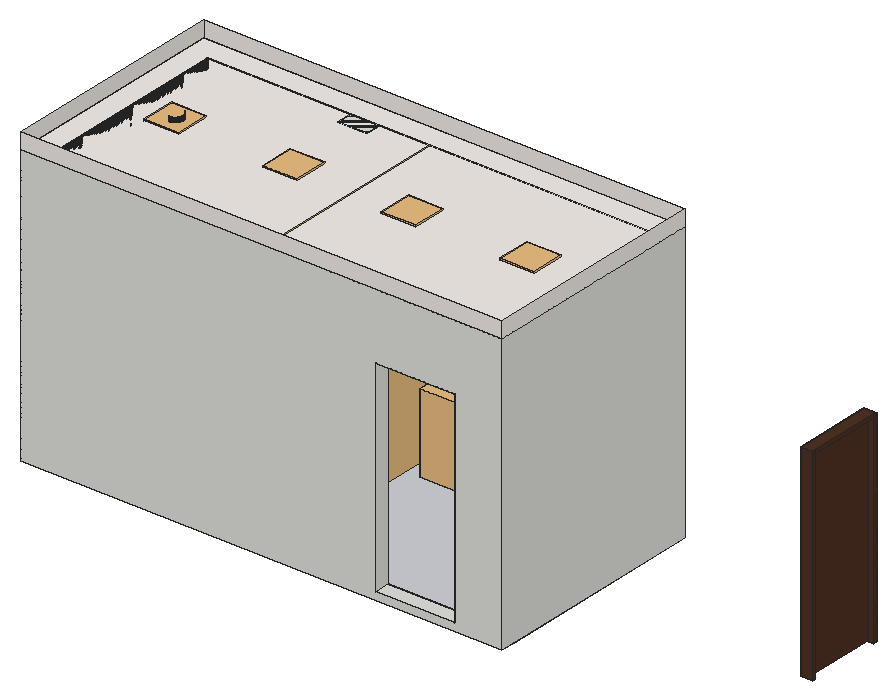
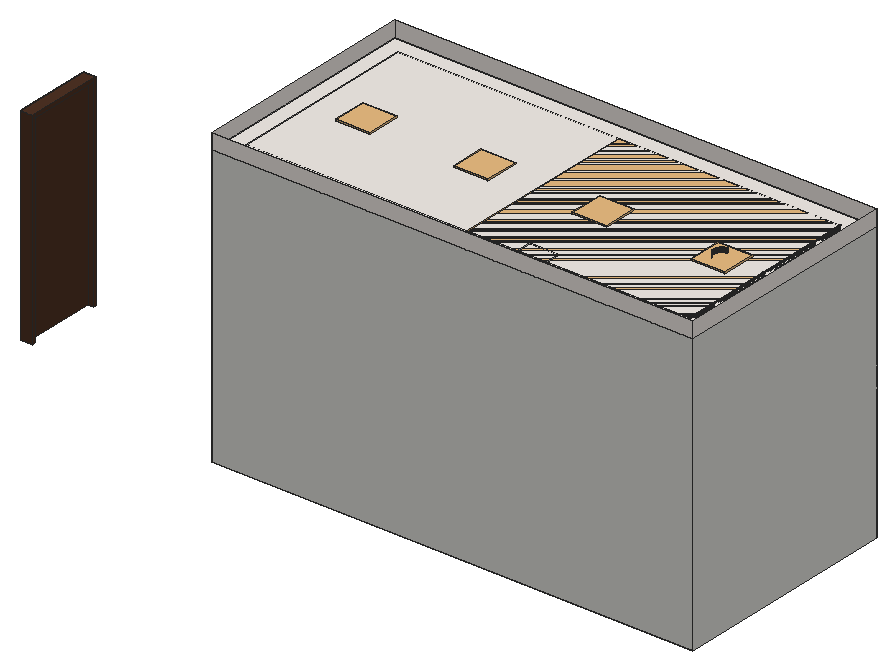
# SketchUp Ruby script. Lengths in inches.
U = 1.inch
M = Sketchup.active_model
def pt(a) = Geom::Point3d.new(a.map { |v| v * U })
def face(e, loops, mat)
  f = e.add_face(loops[0].map { |a| pt(a) })
  loops[1..].each { |l| e.add_face(l.map { |a| pt(a) }).erase! }
  f.material = f.back_material = mat if mat
  f
end
# faces: each face lists its corners as indices into pts; further lists are holes
def faces(e, pts, list, mat = nil) = list.each { |f| face(e, (f[0].is_a?(Array) ? f : [f]).map { |l| l.map { |i| pts[i] } }, mat) }
# xy, xz, yz: faces in a plane at the given z, y or x. An outline is a flat list of corners, or four numbers for a rectangle; further outlines are holes
def ring(l) = l.size == 4 ? [[l[0], l[1]], [l[2], l[1]], [l[2], l[3]], [l[0], l[3]]] : l.each_slice(2).to_a
def flat(e, list, mat, &to3) = list.each { |f| face(e, (f[0].is_a?(Array) ? f : [f]).map { |l| ring(l).map { |u, v| to3.(u, v) } }, mat) }
def xy(e, z, list, mat = nil) = flat(e, list, mat) { |x, y| [x, y, z] }
def xz(e, y, list, mat = nil) = flat(e, list, mat) { |x, z| [x, y, z] }
def yz(e, x, list, mat = nil) = flat(e, list, mat) { |y, z| [x, y, z] }
def lines(e, pts, list) = list.each { |a, b| e.add_line(pt(pts[a]), pt(pts[b])) }
# prism: a flat outline (further loops are holes) pulled along v
def prism(e, loops, v, mat = nil)
  f = face(e, loops, mat); d = Geom::Vector3d.new(v.map { |x| x * U })
  f.pushpull(f.normal.samedirection?(d) ? d.length : -d.length)
end
def box(e, o, s, mat = nil) = prism(e, [[o, [o[0] + s[0], o[1], o[2]], [o[0] + s[0], o[1] + s[1], o[2]], [o[0], o[1] + s[1], o[2]]]], [0, 0, s[2]], mat)
def at(x, y, z, deg = 0) = Geom::Transformation.translation(pt([x, y, z])) * Geom::Transformation.rotation(ORIGIN, Z_AXIS, deg.degrees)
def axes(o, x, y, z) = Geom::Transformation.new([*x, 0, *y, 0, *z, 0, *pt(o).to_a, 1])
def part(name) = M.definitions.add(name)
# library, detail: a bought-in or finely detailed component or shape, given as its bounding box
def library(name, o, s) = part(name).tap { |d| box(d.entities, o, s) }
def detail(e, o, s) = box(e.add_group.entities, o, s)
def put(e, d, t, mat = nil) = e.add_instance(d, t).tap { |i| i.material = mat if mat }
def group(e, t, mat = nil) = e.add_group.tap { |g| g.transformation = t; g.material = mat if mat }.entities
root = M.entities
M.materials.add("0001 AP 9436 AIR BREEZE").color = [243, 237, 232]
M.materials.add("Polis06_194").color = [79, 50, 36]
M.materials.add("Shelves Light").color = [253, 215, 186]
M.materials.add("[Color M00]").color = [255, 255, 255]
M.materials.add("[Marble Carrara Floor Tile]").color = [207, 209, 215]
M.materials.add("[Stone Vein Gray]").color = [234, 229, 229]
M.materials.add("[Terrazzo Tile Light]").color = [219, 217, 210]
c1 = library("Bathrobe with hooks",[0,0,-0.08],[18.125,10.02,52.34])
c2 = library("Bathroom toiletries",[0,-0.3,0],[24.27,4.3,11.74])
c3 = library("Basket & Towel",[-7.51,-8.15,0],[15.02,16.3,23.9375])
c4 = library("JEE-O slimline shower set bronze\#1",[0.04,-0.03,-18.98],[11.61,24.11,65.69])
c5 = library("Group\#4",[-0.25,-72,0],[84.37,72,106])
c6 = part("Difference1")
box(c6.entities,[0,-6,0],[11,6,100])
c7 = part("2")
prism(c7.entities,[[[0.125,0,0],[0.25,0,0],[0.25,0,0.02],[0.25,0,0.03],[0.24,0,0.05],[0.23,0,0.0625],[0.22,0,0.08],[0.21,0,0.09],[0.2,0,0.1],[0.1875,0,0.11],[0.17,0,0.12],[0.16,0,0.12],[0.14,0,0.125],[0.125,0,0.125],[0.11,0,0.125],[0.09,0,0.12],[0.08,0,0.12],[0.0625,0,0.11],[0.05,0,0.1],[0.04,0,0.09],[0.03,0,0.08],[0.02,0,0.0625],[0.01,0,0.05],[0,0,0.03],[0,0,0.02],[0,0,0]]],[0,18,0])
c8 = part("Group\#11")
box(c8.entities,[0,0,0],[17,18,0.125])
g1 = group(c8.entities,at(0,0,0.125))
put(g1,c7,at(2.0625,0,0))
put(g1,c7,at(9.53,0,0))
put(g1,c7,at(10.05,0,0))
put(g1,c7,at(10.57,0,0))
put(g1,c7,at(10.82,0,0))
put(g1,c7,at(5.67,0,0))
put(g1,c7,at(2.32,0,0))
put(g1,c7,at(3.09,0,0))
put(g1,c7,at(1.03,0,0))
put(g1,c7,at(0.77,0,0))
put(g1,c7,at(3.35,0,0))
put(g1,c7,at(5.15,0,0))
put(g1,c7,at(4.38,0,0))
put(g1,c7,at(7.47,0,0))
put(g1,c7,at(8.5,0,0))
put(g1,c7,at(10.31,0,0))
put(g1,c7,at(11.08,0,0))
put(g1,c7,at(2.83,0,0))
put(g1,c7,at(0,0,0))
put(g1,c7,at(1.55,0,0))
put(g1,c7,at(4.125,0,0))
put(g1,c7,at(4.64,0,0))
put(g1,c7,at(4.9,0,0))
put(g1,c7,at(5.41,0,0))
put(g1,c7,at(8.76,0,0))
put(g1,c7,at(3.61,0,0))
put(g1,c7,at(0.52,0,0))
put(g1,c7,at(6.96,0,0))
put(g1,c7,at(7.22,0,0))
put(g1,c7,at(1.29,0,0))
put(g1,c7,at(6.44,0,0))
put(g1,c7,at(7.73,0,0))
put(g1,c7,at(2.58,0,0))
put(g1,c7,at(3.87,0,0))
put(g1,c7,at(6.18,0,0))
put(g1,c7,at(8.25,0,0))
put(g1,c7,at(6.7,0,0))
put(g1,c7,at(9.02,0,0))
put(g1,c7,at(9.79,0,0))
put(g1,c7,at(0.26,0,0))
put(g1,c7,at(1.8,0,0))
put(g1,c7,at(9.28,0,0))
put(g1,c7,at(5.93,0,0))
put(g1,c7,at(7.99,0,0))
put(g1,c7,at(13.92,0,0))
put(g1,c7,at(14.43,0,0))
put(g1,c7,at(14.6875,0,0))
put(g1,c7,at(13.4,0,0))
put(g1,c7,at(12.625,0,0))
put(g1,c7,at(15.98,0,0))
put(g1,c7,at(11.6,0,0))
put(g1,c7,at(11.34,0,0))
put(g1,c7,at(12.88,0,0))
put(g1,c7,at(11.85,0,0))
put(g1,c7,at(13.66,0,0))
put(g1,c7,at(15.2,0,0))
put(g1,c7,at(15.72,0,0))
put(g1,c7,at(14.17,0,0))
put(g1,c7,at(14.95,0,0))
put(g1,c7,at(12.11,0,0))
put(g1,c7,at(12.37,0,0))
put(g1,c7,at(16.23,0,0))
put(g1,c7,at(13.14,0,0))
put(g1,c7,at(16.75,0,0))
put(g1,c7,at(16.49,0,0))
put(g1,c7,at(15.46,0,0))
c9 = part("Group\#9")
put(c9.entities,c8,at(0,0,0.25))
c10 = part("Group\#5")
put(c10.entities,c8,at(0,0,0.25))
c11 = part("Group\#13")
put(c11.entities,c8,at(0,0,0.25))
c12 = library("Group\#22",[0,-21,-2],[57,21,30])
c13 = part("Group\#28")
box(c13.entities,[0,0,-0.5],[18,1,0.5])
c14 = library("Group\#25",[0,-0.44,0],[39,1.19,41])
c15 = part("Bathroom door")
xy(c15.entities,0,[[0,0,4.72,1.18],[0,34.25,4.72,35.43]],"Polis06_194")
xy(c15.entities,85.26,[[0,1.18,4.72,34.25]],"Polis06_194")
xy(c15.entities,86.61,[[0,0,4.72,35.43]],"Polis06_194")
xz(c15.entities,0,[[0,0,4.72,86.61]],"Polis06_194")
xz(c15.entities,1.18,[[0,0,2.36,85.26],[2.36,0,4.72,85.26]],"Polis06_194")
xz(c15.entities,34.25,[[0,0,4.72,85.26]],"Polis06_194")
xz(c15.entities,35.43,[[0,0,4.72,86.61]],"Polis06_194")
yz(c15.entities,0,[[0,0,1.18,86.61],[34.25,0,35.43,86.61],[1.18,85.26,34.25,86.61]],"Polis06_194")
yz(c15.entities,2.36,[[1.18,0,34.25,0,34.25,85.21,1.18,85.26]],"Polis06_194")
yz(c15.entities,4.72,[[0,0,1.18,86.61],[34.25,0,35.43,86.61],[1.18,85.26,34.25,86.61]],"Polis06_194")
c16 = library("Health Faucet",[-0.24,3.23,-9.93],[3.46,9,32.04])
c17 = library("Cesto com toalhas",[0,-0.02,0],[20.47,20.49,27.38])
c18 = library("towels 1",[11.44,13.74,0],[9.37,7.5,4.04])
c19 = library("N_Bathroom Accessory 1",[-8.74,-6.98,-0.07],[10.13,6.73,7.64])
c20 = library("model 1",[0,0,0],[7.72,6.97,5.65])
c21 = library("Plant pots 03",[-13.35,-27.09,0],[26.22,40.73,41.57])
c22 = library("TowelAndHanger",[-0.24,-1.14,-0.4],[8.64,6.67,18.87])
c23 = library("Group\#46",[-1.6,-2.17,0],[14.44,14.68,15.07])
c24 = library("skp31A6",[-6.04,-1.48,32.125],[7.16,7.43,5.2])
c25 = library("Group\#73",[0,0,0],[5.51,2.625,8.11])
c26 = library("_CAPIM_DOS_PAMPAS_JULIAAIRES.3D",[-3.51,-2.78,-196.14],[35.86,35.18,43.25])
c27 = library("Group3\#1",[-226.43,63.68,0],[21.09,21.08,29.58])
c28 = library("15",[-4.61,-4.61,-12.23],[13.01,13.01,12.23])
xy(root,106,[[[0,0,183,87],[68.91,40.5,69.14,40.5,69.22,40.51,69.3,40.51,69.45,40.53,69.53,40.55,69.61,40.5625,69.84,40.62,69.91,40.64,69.99,40.67,70.06,40.69,70.13,40.72,70.21,40.75,70.28,40.79,70.35,40.82,70.42,40.86,70.49,40.89,70.55,40.93,70.62,40.98,70.6875,41.02,70.75,41.0625,70.8125,41.11,71,41.26,71.05,41.3125,71.11,41.37,71.22,41.48,71.42,41.72,71.46,41.79,71.51,41.85,71.59,41.99,71.63,42.05,71.67,42.125,71.7,42.19,71.73,42.26,71.77,42.34,71.79,42.41,71.82,42.48,71.85,42.56,71.87,42.63,71.89,42.71,71.91,42.78,71.93,42.86,71.95,42.9375,71.96,43.01,71.99,43.25,71.99,43.33,72,43.41,72,43.64,71.99,43.72,71.99,43.8,71.97,43.95,71.95,44.03,71.9375,44.11,71.88,44.34,71.86,44.41,71.83,44.49,71.81,44.56,71.78,44.63,71.75,44.71,71.71,44.78,71.68,44.85,71.64,44.92,71.61,44.99,71.57,45.05,71.52,45.12,71.48,45.1875,71.4375,45.25,71.39,45.3125,71.24,45.5,71.1875,45.55,71.13,45.61,71.02,45.72,70.78,45.92,70.71,45.96,70.65,46.01,70.51,46.09,70.45,46.13,70.375,46.17,70.31,46.2,70.24,46.23,70.16,46.27,70.09,46.29,70.02,46.32,69.94,46.35,69.87,46.37,69.79,46.39,69.72,46.41,69.64,46.43,69.5625,46.45,69.49,46.46,69.25,46.49,69.17,46.49,69.09,46.5,68.86,46.5,68.78,46.49,68.7,46.49,68.55,46.47,68.47,46.45,68.39,46.4375,68.16,46.38,68.09,46.36,68.01,46.33,67.94,46.31,67.87,46.28,67.79,46.25,67.72,46.21,67.65,46.18,67.58,46.14,67.51,46.11,67.45,46.07,67.38,46.02,67.3125,45.98,67.25,45.9375,67.1875,45.89,67,45.74,66.95,45.6875,66.89,45.63,66.78,45.52,66.58,45.28,66.54,45.21,66.49,45.15,66.41,45.01,66.37,44.95,66.33,44.875,66.3,44.81,66.27,44.74,66.23,44.66,66.21,44.59,66.18,44.52,66.15,44.44,66.13,44.37,66.11,44.29,66.09,44.22,66.07,44.14,66.05,44.0625,66.04,43.99,66.01,43.75,66.01,43.67,66,43.59,66,43.36,66.01,43.28,66.01,43.2,66.03,43.05,66.05,42.97,66.0625,42.89,66.12,42.66,66.14,42.59,66.17,42.51,66.19,42.44,66.22,42.37,66.25,42.29,66.29,42.22,66.32,42.15,66.36,42.08,66.39,42.01,66.43,41.95,66.48,41.88,66.52,41.8125,66.5625,41.75,66.61,41.6875,66.76,41.5,66.8125,41.45,66.87,41.39,66.98,41.28,67.22,41.08,67.29,41.04,67.35,40.99,67.49,40.91,67.55,40.87,67.625,40.83,67.69,40.8,67.76,40.77,67.84,40.73,67.91,40.71,67.98,40.68,68.06,40.65,68.13,40.63,68.21,40.61,68.28,40.59,68.36,40.57,68.4375,40.55,68.51,40.54,68.75,40.51,68.83,40.51],[23.91,40.5,24.14,40.5,24.22,40.51,24.3,40.51,24.45,40.53,24.53,40.55,24.61,40.5625,24.84,40.62,24.91,40.64,24.99,40.67,25.06,40.69,25.13,40.72,25.21,40.75,25.28,40.79,25.35,40.82,25.42,40.86,25.49,40.89,25.55,40.93,25.62,40.98,25.6875,41.02,25.75,41.0625,25.8125,41.11,26,41.26,26.05,41.3125,26.11,41.37,26.22,41.48,26.42,41.72,26.46,41.79,26.51,41.85,26.59,41.99,26.63,42.05,26.67,42.125,26.7,42.19,26.73,42.26,26.77,42.34,26.79,42.41,26.82,42.48,26.85,42.56,26.87,42.63,26.89,42.71,26.91,42.78,26.93,42.86,26.95,42.9375,26.96,43.01,26.99,43.25,26.99,43.33,27,43.41,27,43.64,26.99,43.72,26.99,43.8,26.97,43.95,26.95,44.03,26.9375,44.11,26.88,44.34,26.86,44.41,26.83,44.49,26.81,44.56,26.78,44.63,26.75,44.71,26.71,44.78,26.68,44.85,26.64,44.92,26.61,44.99,26.57,45.05,26.52,45.12,26.48,45.1875,26.4375,45.25,26.39,45.3125,26.24,45.5,26.1875,45.55,26.13,45.61,26.02,45.72,25.78,45.92,25.71,45.96,25.65,46.01,25.51,46.09,25.45,46.13,25.375,46.17,25.31,46.2,25.24,46.23,25.16,46.27,25.09,46.29,25.02,46.32,24.94,46.35,24.87,46.37,24.79,46.39,24.72,46.41,24.64,46.43,24.5625,46.45,24.49,46.46,24.25,46.49,24.17,46.49,24.09,46.5,23.86,46.5,23.78,46.49,23.7,46.49,23.55,46.47,23.47,46.45,23.39,46.4375,23.16,46.38,23.09,46.36,23.01,46.33,22.94,46.31,22.87,46.28,22.79,46.25,22.72,46.21,22.65,46.18,22.58,46.14,22.51,46.11,22.45,46.07,22.38,46.02,22.3125,45.98,22.25,45.9375,22.1875,45.89,22,45.74,21.95,45.6875,21.89,45.63,21.78,45.52,21.58,45.28,21.54,45.21,21.49,45.15,21.41,45.01,21.37,44.95,21.33,44.875,21.3,44.81,21.27,44.74,21.23,44.66,21.21,44.59,21.18,44.52,21.15,44.44,21.13,44.37,21.11,44.29,21.09,44.22,21.07,44.14,21.05,44.0625,21.04,43.99,21.01,43.75,21.01,43.67,21,43.59,21,43.36,21.01,43.28,21.01,43.2,21.03,43.05,21.05,42.97,21.0625,42.89,21.12,42.66,21.14,42.59,21.17,42.51,21.19,42.44,21.22,42.37,21.25,42.29,21.29,42.22,21.32,42.15,21.36,42.08,21.39,42.01,21.43,41.95,21.48,41.88,21.52,41.8125,21.5625,41.75,21.61,41.6875,21.76,41.5,21.8125,41.45,21.87,41.39,21.98,41.28,22.22,41.08,22.29,41.04,22.35,40.99,22.49,40.91,22.55,40.87,22.625,40.83,22.69,40.8,22.76,40.77,22.84,40.73,22.91,40.71,22.98,40.68,23.06,40.65,23.13,40.63,23.21,40.61,23.28,40.59,23.36,40.57,23.4375,40.55,23.51,40.54,23.75,40.51,23.83,40.51],[158.91,40.5,159.14,40.5,159.22,40.51,159.3,40.51,159.45,40.53,159.53,40.55,159.61,40.5625,159.84,40.62,159.91,40.64,159.99,40.67,160.06,40.69,160.13,40.72,160.21,40.75,160.28,40.79,160.35,40.82,160.42,40.86,160.49,40.89,160.55,40.93,160.62,40.98,160.6875,41.02,160.75,41.0625,160.8125,41.11,161,41.26,161.05,41.3125,161.11,41.37,161.22,41.48,161.42,41.72,161.46,41.79,161.51,41.85,161.59,41.99,161.63,42.05,161.67,42.125,161.7,42.19,161.73,42.26,161.77,42.34,161.79,42.41,161.82,42.48,161.85,42.56,161.87,42.63,161.89,42.71,161.91,42.78,161.93,42.86,161.95,42.9375,161.96,43.01,161.99,43.25,161.99,43.33,162,43.41,162,43.64,161.99,43.72,161.99,43.8,161.97,43.95,161.95,44.03,161.9375,44.11,161.88,44.34,161.86,44.41,161.83,44.49,161.81,44.56,161.78,44.63,161.75,44.71,161.71,44.78,161.68,44.85,161.64,44.92,161.61,44.99,161.57,45.05,161.52,45.12,161.48,45.1875,161.4375,45.25,161.39,45.3125,161.24,45.5,161.1875,45.55,161.13,45.61,161.02,45.72,160.78,45.92,160.71,45.96,160.65,46.01,160.51,46.09,160.45,46.13,160.375,46.17,160.31,46.2,160.24,46.23,160.16,46.27,160.09,46.29,160.02,46.32,159.94,46.35,159.87,46.37,159.79,46.39,159.72,46.41,159.64,46.43,159.5625,46.45,159.49,46.46,159.25,46.49,159.17,46.49,159.09,46.5,158.86,46.5,158.78,46.49,158.7,46.49,158.55,46.47,158.47,46.45,158.39,46.4375,158.16,46.38,158.09,46.36,158.01,46.33,157.94,46.31,157.87,46.28,157.79,46.25,157.72,46.21,157.65,46.18,157.58,46.14,157.51,46.11,157.45,46.07,157.38,46.02,157.3125,45.98,157.25,45.9375,157.1875,45.89,157,45.74,156.95,45.6875,156.89,45.63,156.78,45.52,156.58,45.28,156.54,45.21,156.49,45.15,156.41,45.01,156.37,44.95,156.33,44.875,156.3,44.81,156.27,44.74,156.23,44.66,156.21,44.59,156.18,44.52,156.15,44.44,156.13,44.37,156.11,44.29,156.09,44.22,156.07,44.14,156.05,44.0625,156.04,43.99,156.01,43.75,156.01,43.67,156,43.59,156,43.36,156.01,43.28,156.01,43.2,156.03,43.05,156.05,42.97,156.0625,42.89,156.12,42.66,156.14,42.59,156.17,42.51,156.19,42.44,156.22,42.37,156.25,42.29,156.29,42.22,156.32,42.15,156.36,42.08,156.39,42.01,156.43,41.95,156.48,41.88,156.52,41.8125,156.5625,41.75,156.61,41.6875,156.76,41.5,156.8125,41.45,156.87,41.39,156.98,41.28,157.22,41.08,157.29,41.04,157.35,40.99,157.49,40.91,157.55,40.87,157.625,40.83,157.69,40.8,157.76,40.77,157.84,40.73,157.91,40.71,157.98,40.68,158.06,40.65,158.13,40.63,158.21,40.61,158.28,40.59,158.36,40.57,158.4375,40.55,158.51,40.54,158.75,40.51,158.83,40.51],[113.91,40.5,114.14,40.5,114.22,40.51,114.3,40.51,114.45,40.53,114.53,40.55,114.61,40.5625,114.84,40.62,114.91,40.64,114.99,40.67,115.06,40.69,115.13,40.72,115.21,40.75,115.28,40.79,115.35,40.82,115.42,40.86,115.49,40.89,115.55,40.93,115.62,40.98,115.6875,41.02,115.75,41.0625,115.8125,41.11,116,41.26,116.05,41.3125,116.11,41.37,116.22,41.48,116.42,41.72,116.46,41.79,116.51,41.85,116.59,41.99,116.63,42.05,116.67,42.125,116.7,42.19,116.73,42.26,116.77,42.34,116.79,42.41,116.82,42.48,116.85,42.56,116.87,42.63,116.89,42.71,116.91,42.78,116.93,42.86,116.95,42.9375,116.96,43.01,116.99,43.25,116.99,43.33,117,43.41,117,43.64,116.99,43.72,116.99,43.8,116.97,43.95,116.95,44.03,116.9375,44.11,116.88,44.34,116.86,44.41,116.83,44.49,116.81,44.56,116.78,44.63,116.75,44.71,116.71,44.78,116.68,44.85,116.64,44.92,116.61,44.99,116.57,45.05,116.52,45.12,116.48,45.1875,116.4375,45.25,116.39,45.3125,116.24,45.5,116.1875,45.55,116.13,45.61,116.02,45.72,115.78,45.92,115.71,45.96,115.65,46.01,115.51,46.09,115.45,46.13,115.375,46.17,115.31,46.2,115.24,46.23,115.16,46.27,115.09,46.29,115.02,46.32,114.94,46.35,114.87,46.37,114.79,46.39,114.72,46.41,114.64,46.43,114.5625,46.45,114.49,46.46,114.25,46.49,114.17,46.49,114.09,46.5,113.86,46.5,113.78,46.49,113.7,46.49,113.55,46.47,113.47,46.45,113.39,46.4375,113.16,46.38,113.09,46.36,113.01,46.33,112.94,46.31,112.87,46.28,112.79,46.25,112.72,46.21,112.65,46.18,112.58,46.14,112.51,46.11,112.45,46.07,112.38,46.02,112.3125,45.98,112.25,45.9375,112.1875,45.89,112,45.74,111.95,45.6875,111.89,45.63,111.78,45.52,111.58,45.28,111.54,45.21,111.49,45.15,111.41,45.01,111.37,44.95,111.33,44.875,111.3,44.81,111.27,44.74,111.23,44.66,111.21,44.59,111.18,44.52,111.15,44.44,111.13,44.37,111.11,44.29,111.09,44.22,111.07,44.14,111.05,44.0625,111.04,43.99,111.01,43.75,111.01,43.67,111,43.59,111,43.36,111.01,43.28,111.01,43.2,111.03,43.05,111.05,42.97,111.0625,42.89,111.12,42.66,111.14,42.59,111.17,42.51,111.19,42.44,111.22,42.37,111.25,42.29,111.29,42.22,111.32,42.15,111.36,42.08,111.39,42.01,111.43,41.95,111.48,41.88,111.52,41.8125,111.5625,41.75,111.61,41.6875,111.76,41.5,111.8125,41.45,111.87,41.39,111.98,41.28,112.22,41.08,112.29,41.04,112.35,40.99,112.49,40.91,112.55,40.87,112.625,40.83,112.69,40.8,112.76,40.77,112.84,40.73,112.91,40.71,112.98,40.68,113.06,40.65,113.13,40.63,113.21,40.61,113.28,40.59,113.36,40.57,113.4375,40.55,113.51,40.54,113.75,40.51,113.83,40.51]]],"0001 AP 9436 AIR BREEZE")
xz(root,0,[[0,106,183,112]],"0001 AP 9436 AIR BREEZE")
xz(root,40.5,[[23.91,106,23.98,108],[23.98,106,24.0625,108],[24.0625,106,24.14,108]],"0001 AP 9436 AIR BREEZE")
xz(root,40.51,[[24.22,106,24.3,108]],"0001 AP 9436 AIR BREEZE")
xz(root,87,[[0,106,183,112]],"0001 AP 9436 AIR BREEZE")
yz(root,0,[[0,106,87,112]],"0001 AP 9436 AIR BREEZE")
yz(root,26.99,[[43.25,106,43.33,108],[43.72,106,43.8,108]],"0001 AP 9436 AIR BREEZE")
yz(root,27,[[43.41,106,43.48,108],[43.48,106,43.5625,108],[43.5625,106,43.64,108]],"0001 AP 9436 AIR BREEZE")
yz(root,183,[[0,106,87,112]],"0001 AP 9436 AIR BREEZE")
p = [[24.22,40.51,106],[24.14,40.5,106],[24.14,40.5,108],[24.22,40.51,108],[24.375,40.52,106],[24.3,40.51,106],
  [24.3,40.51,108],[24.375,40.52,108],[24.45,40.53,106],[24.45,40.53,108],[24.61,40.5625,106],[24.53,40.55,106],
  [24.53,40.55,108],[24.61,40.5625,108],[24.68,40.58,106],[24.68,40.58,108],[24.76,40.6,106],[24.76,40.6,108],
  [24.91,40.64,106],[24.84,40.62,106],[24.84,40.62,108],[24.91,40.64,108],[24.99,40.67,106],[24.99,40.67,108],
  [25.06,40.69,106],[25.06,40.69,108],[25.21,40.75,106],[25.13,40.72,106],[25.13,40.72,108],[25.21,40.75,108],
  [25.28,40.79,106],[25.28,40.79,108],[25.42,40.86,106],[25.35,40.82,106],[25.35,40.82,108],[25.42,40.86,108],
  [25.49,40.89,106],[25.49,40.89,108],[25.55,40.93,106],[25.55,40.93,108],[25.62,40.98,106],[25.62,40.98,108],
  [25.6875,41.02,106],[25.6875,41.02,108],[25.75,41.0625,106],[25.75,41.0625,108],[25.875,41.16,106],[25.8125,41.11,106],
  [25.8125,41.11,108],[25.875,41.16,108],[26,41.26,106],[25.9375,41.21,106],[25.9375,41.21,108],[26,41.26,108],
  [26.05,41.3125,106],[26.05,41.3125,108],[26.11,41.37,106],[26.11,41.37,108],[26.16,41.42,106],[26.16,41.42,108],
  [26.22,41.48,106],[26.22,41.48,108],[26.27,41.54,106],[26.27,41.54,108],[26.32,41.6,106],[26.32,41.6,108],
  [26.37,41.66,106],[26.37,41.66,108],[26.46,41.79,106],[26.42,41.72,106],[26.42,41.72,108],[26.46,41.79,108],
  [26.51,41.85,106],[26.51,41.85,108],[26.59,41.99,106],[26.55,41.92,106],[26.55,41.92,108],[26.59,41.99,108],
  [26.63,42.05,106],[26.63,42.05,108],[26.67,42.125,106],[26.67,42.125,108],[26.7,42.19,106],[26.7,42.19,108],
  [26.73,42.26,106],[26.73,42.26,108],[26.77,42.34,106],[26.77,42.34,108],[26.79,42.41,106],[26.79,42.41,108],
  [26.82,42.48,106],[26.82,42.48,108],[26.85,42.56,106],[26.85,42.56,108],[26.87,42.63,106],[26.87,42.63,108],
  [26.89,42.71,106],[26.89,42.71,108],[26.91,42.78,106],[26.91,42.78,108],[26.93,42.86,106],[26.93,42.86,108],
  [26.96,43.01,106],[26.95,42.9375,106],[26.95,42.9375,108],[26.96,43.01,108],[26.97,43.09,106],[26.97,43.09,108],
  [26.98,43.17,106],[26.98,43.17,108],[26.99,43.25,106],[26.99,43.25,108],[27,43.41,106],[26.99,43.33,106],
  [26.99,43.33,108],[27,43.41,108],[26.99,43.72,106],[27,43.64,106],[27,43.64,108],[26.99,43.72,108],
  [26.98,43.875,106],[26.99,43.8,106],[26.99,43.8,108],[26.98,43.875,108],[26.97,43.95,106],[26.97,43.95,108],
  [26.9375,44.11,106],[26.95,44.03,106],[26.95,44.03,108],[26.9375,44.11,108],[26.92,44.18,106],[26.92,44.18,108],
  [26.9,44.26,106],[26.9,44.26,108],[26.86,44.41,106],[26.88,44.34,106],[26.88,44.34,108],[26.86,44.41,108],
  [26.83,44.49,106],[26.83,44.49,108],[26.81,44.56,106],[26.81,44.56,108],[26.75,44.71,106],[26.78,44.63,106],
  [26.78,44.63,108],[26.75,44.71,108],[26.71,44.78,106],[26.71,44.78,108],[26.64,44.92,106],[26.68,44.85,106],
  [26.68,44.85,108],[26.64,44.92,108],[26.61,44.99,106],[26.61,44.99,108],[26.57,45.05,106],[26.57,45.05,108],
  [26.48,45.1875,106],[26.52,45.12,106],[26.52,45.12,108],[26.48,45.1875,108],[26.4375,45.25,106],[26.4375,45.25,108],
  [26.34,45.375,106],[26.39,45.3125,106],[26.39,45.3125,108],[26.34,45.375,108],[26.24,45.5,106],[26.29,45.4375,106],
  [26.29,45.4375,108],[26.24,45.5,108],[26.1875,45.55,106],[26.1875,45.55,108],[26.08,45.66,106],[26.13,45.61,106],
  [26.13,45.61,108],[26.08,45.66,108],[25.96,45.77,106],[26.02,45.72,106],[26.02,45.72,108],[25.96,45.77,108],
  [25.84,45.87,106],[25.9,45.82,106],[25.9,45.82,108],[25.84,45.87,108],[25.78,45.92,106],[25.78,45.92,108]]
faces(root,p,[[0,1,2,3],[4,5,6,7],[8,4,7,9],[10,11,12,13],[11,8,9,12],[14,10,13,15],[16,14,15,17],[18,19,20,21],
  [19,16,17,20],[22,18,21,23],[24,22,23,25],[26,27,28,29],[27,24,25,28],[30,26,29,31],[32,33,34,35],[33,30,31,34],
  [36,32,35,37],[38,36,37,39],[40,38,39,41],[42,40,41,43],[44,42,43,45],[46,47,48,49],[47,44,45,48],[50,51,52,53],
  [51,46,49,52],[54,50,53,55],[56,54,55,57],[58,56,57,59],[60,58,59,61],[62,60,61,63],[64,62,63,65],[66,64,65,67],
  [68,69,70,71],[69,66,67,70],[72,68,71,73],[74,75,76,77],[75,72,73,76],[78,74,77,79],[80,78,79,81],[82,80,81,83],
  [84,82,83,85],[86,84,85,87],[88,86,87,89],[90,88,89,91],[92,90,91,93],[94,92,93,95],[96,94,95,97],[98,96,97,99],
  [100,98,99,101],[102,103,104,105],[103,100,101,104],[106,102,105,107],[108,106,107,109],[110,108,109,111],[112,113,114,115],[116,117,118,119],
  [120,121,122,123],[124,120,123,125],[126,127,128,129],[127,124,125,128],[130,126,129,131],[132,130,131,133],[134,135,136,137],[135,132,133,136],
  [138,134,137,139],[140,138,139,141],[142,143,144,145],[143,140,141,144],[146,142,145,147],[148,149,150,151],[149,146,147,150],[152,148,151,153],
  [154,152,153,155],[156,157,158,159],[157,154,155,158],[160,156,159,161],[162,163,164,165],[163,160,161,164],[166,167,168,169],[167,162,165,168],
  [170,166,169,171],[172,173,174,175],[173,170,171,174],[176,177,178,179],[177,172,175,178],[180,181,182,183],[181,176,179,182],[184,180,183,185]],"0001 AP 9436 AIR BREEZE")
g2 = group(root,at(3,6,0))
xy(g2,0,[[-3,-6,-3,81,180,81,180,0,174,0,174,72,5.75,72,5.75,0,180,0,180,-6]])
xy(g2,3,[[132,-6,162,0]])
xy(g2,42,[[71,71,91,72]],"0001 AP 9436 AIR BREEZE")
xy(g2,43,[[72,71,90,76.5]],"0001 AP 9436 AIR BREEZE")
xy(g2,46,[[2.5,12,5.75,60]],"0001 AP 9436 AIR BREEZE")
xy(g2,56.83,[[72,71,90,75.5]])
xy(g2,57.33,[[72,75.5,90,76.5]])
xy(g2,57.83,[[72,71,90,76.5]],"0001 AP 9436 AIR BREEZE")
xy(g2,64,[[3,12,5.75,60]],"0001 AP 9436 AIR BREEZE")
xy(g2,64.5,[[2.5,12,3,60]])
xy(g2,71.17,[[72,71,90,75.5]])
xy(g2,71.67,[[72,75.5,90,76.5]])
xy(g2,72.17,[[72,71,90,76.5]],"0001 AP 9436 AIR BREEZE")
xy(g2,81,[[132,-6,162,0]])
xy(g2,86,[[72,71,90,75.5]])
xy(g2,86.5,[[72,75.5,90,76.5]])
xy(g2,87,[[71,71,91,72]],"0001 AP 9436 AIR BREEZE")
xy(g2,106,[[[-3,-6,180,81],[5.75,0,174,72]]])
xz(g2,-6,[[[-3,0,180,106],[132,3,162,81]]])
xz(g2,0,[[[5.75,0,174,106],[132,3,162,81]]])
xz(g2,12,[[2.5,46,2.5,64.5,3,64.5,3,64,5.75,64,5.75,46]])
xz(g2,60,[[2.5,46,5.75,46,5.75,64,3,64,3,64.5,2.5,64.5]],"0001 AP 9436 AIR BREEZE")
xz(g2,71,[[[71,42,91,87],[72,72.17,90,86],[72,43,90,56.83],[72,57.83,90,71.17]]],"0001 AP 9436 AIR BREEZE")
xz(g2,72,[[[60,0,174,106],[71,42,91,87]]],"0001 AP 9436 AIR BREEZE")
xz(g2,72,[[5.75,0,60,106]],"[Stone Vein Gray]")
xz(g2,75.5,[[72,56.83,90,57.33],[72,71.17,90,71.67],[72,86,90,86.5]])
xz(g2,76.5,[[72,43,90,57.33],[72,57.83,90,71.67],[72,72.17,90,86.5]])
xz(g2,81,[[-3,0,180,106]])
yz(g2,-3,[[-6,0,81,106]])
yz(g2,2.5,[[12,46,60,64.5]],"0001 AP 9436 AIR BREEZE")
yz(g2,3,[[12,64,60,64.5]])
yz(g2,5.75,[[[0,0,72,106],[12,46,60,64]]])
yz(g2,71,[[71,42,72,87]])
yz(g2,72,[[71,43,76.5,43,76.5,57.33,75.5,57.33,75.5,56.83,71,56.83],[71,57.83,76.5,57.83,76.5,71.67,75.5,71.67,75.5,71.17,71,71.17],[71,72.17,76.5,72.17,76.5,86.5,75.5,86.5,75.5,86,71,86]],"0001 AP 9436 AIR BREEZE")
yz(g2,90,[[71,43,71,56.83,75.5,56.83,75.5,57.33,76.5,57.33,76.5,43],[71,57.83,71,71.17,75.5,71.17,75.5,71.67,76.5,71.67,76.5,57.83],[71,72.17,71,86,75.5,86,75.5,86.5,76.5,86.5,76.5,72.17]],"0001 AP 9436 AIR BREEZE")
yz(g2,91,[[71,42,72,87]],"0001 AP 9436 AIR BREEZE")
yz(g2,132,[[-6,3,0,81]])
yz(g2,162,[[-6,3,0,81]])
yz(g2,174,[[0,0,72,106]],"0001 AP 9436 AIR BREEZE")
yz(g2,180,[[-6,0,81,106]])
put(g2,c1,at(174,19.1,24.54,90))
put(g2,c2,axes([5.66,35.73,46.11],[0,1,0],[-0.70602,0,0],[0,0,0.86]))
put(g2,c3,at(165.61,40.65,0))
put(g2,c4,at(26.65,47.92,36.18))
put(g2,c5,at(6,72,0))
put(g2,c6,axes([60,72,0],[1,0,0],[0,1,0],[0,0,1.06]))
g3 = group(g2,at(5.75,0,4),"[Terrazzo Tile Light]")
put(g3,c9,axes([-0.25,36,42],[0,0,-1.24059],[0,1.33333,0],[1,0,0]))
put(g3,c9,axes([-0.25,12,42],[0,0,-1.24059],[0,1.33333,0],[1,0,0]))
put(g3,c10,axes([-0.25,36,20.91],[0,0,-1.23],[0,1.33333,0],[1,0,0]))
put(g3,c10,axes([-0.25,12,20.91],[0,0,-1.23],[0,1.33333,0],[1,0,0]))
g4 = group(g3,at(-0.25,36,80.9375))
put(g4,c8,axes([0.25,0,0],[0,0,-1.23152],[0,1.33333,0],[1,0,0]))
put(g3,c9,axes([-0.25,36,102.05],[0,0,-1.2423],[0,1.33333,0],[1,0,0]))
g5 = group(g3,at(-0.25,12,102.05))
put(g5,c8,axes([0.25,0,0],[0,0,-1.2423],[0,1.33333,0],[1,0,0]))
put(g3,c10,axes([-0.25,12,80.9375],[0,0,-1.23152],[0,1.33333,0],[1,0,0]))
put(g3,c10,axes([-0.25,60,17],[0,0,-1],[0,0.66667,0],[1,0,0]))
put(g3,c11,axes([-0.25,60,85],[0,0,-1],[0,0.66667,0],[1,0,0]))
put(g3,c11,axes([-0.25,60,68],[0,0,-1],[0,0.66667,0],[1,0,0]))
put(g3,c9,axes([-0.25,60,34],[0,0,-1],[0,0.66667,0],[1,0,0]))
put(g3,c11,axes([-0.25,60,51],[0,0,-1],[0,0.66667,0],[1,0,0]))
put(g3,c11,axes([-0.25,60,102],[0,0,-1],[0,0.66667,0],[1,0,0]))
put(g3,c11,axes([-0.25,12,85],[0,0,-1],[0,-0.66667,0],[1,0,0]))
put(g3,c11,axes([-0.25,12,68],[0,0,-1],[0,-0.66667,0],[1,0,0]))
put(g3,c9,axes([-0.25,12,34],[0,0,-1],[0,-0.66667,0],[1,0,0]))
put(g3,c11,axes([-0.25,12,51],[0,0,-1],[0,-0.66667,0],[1,0,0]))
put(g3,c11,axes([-0.25,12,102],[0,0,-1],[0,-0.66667,0],[1,0,0]))
put(g3,c10,axes([-0.25,12,17],[0,0,-1],[0,-0.66667,0],[1,0,0]))
put(g2,c12,at(103,72,9))
g6 = group(g2,at(160,72,7),"0001 AP 9436 AIR BREEZE")
xy(g6,0,[[0,-18,14,0]])
xy(g6,1,[[1,-18,13,-1]])
xy(g6,15.67,[[1,-18,13,-2]])
xy(g6,16.17,[[1,-2,13,-1]])
xy(g6,16.67,[[1,-18,13,-1]])
xy(g6,30.83,[[1,-18,13,-2]])
xy(g6,31.33,[[1,-2,13,-1]])
xy(g6,31.83,[[1,-18,13,-1]])
xy(g6,46,[[1,-18,13,-2]])
xy(g6,46.5,[[1,-2,13,-1]])
xy(g6,47,[[1,-18,13,-1]])
xy(g6,61.17,[[1,-18,13,-2]])
xy(g6,61.67,[[1,-2,13,-1]])
xy(g6,62.17,[[1,-18,13,-1]])
xy(g6,76.33,[[1,-18,13,-2]])
xy(g6,76.83,[[1,-2,13,-1]])
xy(g6,77.33,[[1,-18,13,-1]])
xy(g6,92,[[1,-18,13,-2]])
xy(g6,92.5,[[1,-2,13,-1]])
xy(g6,93,[[0,-18,14,0]])
xz(g6,-18,[[[0,0,14,93],[1,77.33,13,92],[1,1,13,15.67],[1,31.83,13,46],[1,47,13,61.17],[1,16.67,13,30.83],[1,62.17,13,76.33]]])
xz(g6,-2,[[1,15.67,13,16.17],[1,30.83,13,31.33],[1,46,13,46.5],[1,61.17,13,61.67],[1,76.33,13,76.83],
  [1,92,13,92.5]])
xz(g6,-1,[[1,1,13,16.17],[1,16.67,13,31.33],[1,31.83,13,46.5],[1,47,13,61.67],[1,62.17,13,76.83],
  [1,77.33,13,92.5]])
xz(g6,0,[[0,0,14,93]])
yz(g6,0,[[-18,0,0,93]])
yz(g6,1,[[-18,1,-1,1,-1,16.17,-2,16.17,-2,15.67,-18,15.67],[-18,16.67,-1,16.67,-1,31.33,-2,31.33,-2,30.83,-18,30.83],[-18,31.83,-1,31.83,-1,46.5,-2,46.5,-2,46,-18,46],[-18,47,-1,47,-1,61.67,-2,61.67,-2,61.17,-18,61.17],[-18,62.17,-1,62.17,-1,76.83,-2,76.83,-2,76.33,-18,76.33],
  [-18,77.33,-1,77.33,-1,92.5,-2,92.5,-2,92,-18,92]])
yz(g6,13,[[-18,1,-18,15.67,-2,15.67,-2,16.17,-1,16.17,-1,1],[-18,16.67,-18,30.83,-2,30.83,-2,31.33,-1,31.33,-1,16.67],[-18,31.83,-18,46,-2,46,-2,46.5,-1,46.5,-1,31.83],[-18,47,-18,61.17,-2,61.17,-2,61.67,-1,61.67,-1,47],[-18,62.17,-18,76.33,-2,76.33,-2,76.83,-1,76.83,-1,62.17],
  [-18,77.33,-18,92,-2,92,-2,92.5,-1,92.5,-1,77.33]])
yz(g6,14,[[-18,0,0,93]])
put(g6,c13,axes([1,-2,16.17],[0.66667,0,0],[0,1,0],[0,0,1]),"Shelves Light")
put(g6,c13,axes([1,-2,31.33],[0.66667,0,0],[0,1,0],[0,0,1]),"Shelves Light")
put(g6,c13,axes([1,-2,46.5],[0.66667,0,0],[0,1,0],[0,0,1]),"Shelves Light")
put(g6,c13,axes([1,-2,61.67],[0.66667,0,0],[0,1,0],[0,0,1]),"Shelves Light")
put(g6,c13,axes([1,-2,76.83],[0.66667,0,0],[0,1,0],[0,0,1]),"Shelves Light")
put(g6,c13,axes([1,-2,92.5],[0.66667,0,0],[0,1,0],[0,0,1]),"Shelves Light")
put(g2,c14,at(112,71.25,46))
put(g2,c13,at(72,75.5,57.33),"Shelves Light")
put(g2,c13,at(72,75.5,71.67),"Shelves Light")
put(g2,c13,at(72,75.5,86.5),"Shelves Light")
put(g2,c13,axes([3,12,64.5],[0,2.66667,0],[-0.5,0,0],[0,0,1]),"Shelves Light")
g7 = group(root,at(9,6,0),"[Marble Carrara Floor Tile]")
box(g7,[0,0,0],[168,72,0.1])
put(root,c15,axes([265.28,39,3],[1,0,0],[0,0.84667,0],[0,0,0.90055]))
put(root,c16,at(63.9375,71.76,14.2,-90))
put(root,c17,axes([165.44,69.47,8],[0,-0.4625,0],[0.4625,0,0],[0,0,0.4625]))
put(root,c18,at(153.57,47.99,23.67))
put(root,c19,at(160.93,73.66,37))
put(root,c20,at(115.26,73.79,37,-180))
put(root,c21,axes([173.11,65.62,38.83],[0,-0.3,0],[0.3,0,0],[0,0,0.3]))
put(root,c21,axes([86.18,79.18,43],[0,-0.3,0],[0.3,0,0],[0,0,0.3]))
put(root,c22,at(100.52,73.93,43.97))
put(root,c23,axes([4.82,24.25,46],[0,-0.47,0],[0.47,0,0],[0,0,0.47]))
put(root,c24,at(172.84,63.31,21.875))
put(root,c25,axes([82.41,77,57.83],[1.49,0,0],[0,1.49,0],[0,0,1.49]))
put(root,c24,at(172.84,63.31,37.04))
put(root,c26,axes([73.96,83.09,132.97],[0,-0.31,0],[0.31,0,0],[0,0,0.31]))
put(root,c27,axes([147.09,2.11,84.33],[0,-0.3,0],[0.3,0,0],[0,0,0.3]))
put(root,c28,at(22.11,41.61,106.375),"0001 AP 9436 AIR BREEZE")
put(root,c28,at(67.11,41.61,106.375),"0001 AP 9436 AIR BREEZE")
put(root,c28,at(112.11,41.61,106.375),"[Color M00]")
put(root,c28,at(157.11,41.61,106.375),"0001 AP 9436 AIR BREEZE")
